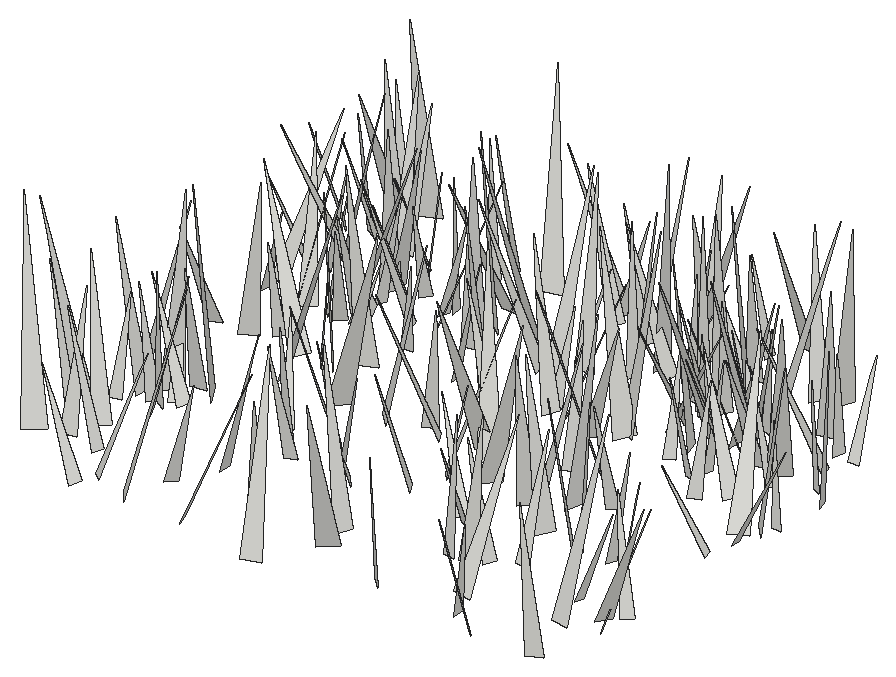
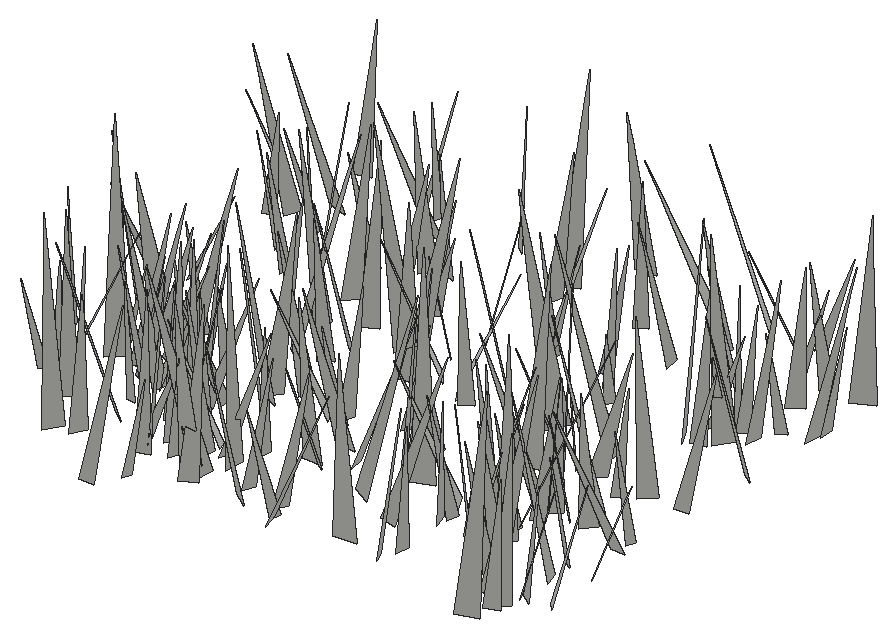
# SketchUp Ruby script. Lengths in inches.
U = 1.inch
M = Sketchup.active_model
def pt(a) = Geom::Point3d.new(a.map { |v| v * U })
def face(e, loops, mat)
  f = e.add_face(loops[0].map { |a| pt(a) })
  loops[1..].each { |l| e.add_face(l.map { |a| pt(a) }).erase! }
  f.material = f.back_material = mat if mat
  f
end
# faces: each face lists its corners as indices into pts; further lists are holes
def faces(e, pts, list, mat = nil) = list.each { |f| face(e, (f[0].is_a?(Array) ? f : [f]).map { |l| l.map { |i| pts[i] } }, mat) }
# xy, xz, yz: faces in a plane at the given z, y or x. An outline is a flat list of corners, or four numbers for a rectangle; further outlines are holes
def ring(l) = l.size == 4 ? [[l[0], l[1]], [l[2], l[1]], [l[2], l[3]], [l[0], l[3]]] : l.each_slice(2).to_a
def flat(e, list, mat, &to3) = list.each { |f| face(e, (f[0].is_a?(Array) ? f : [f]).map { |l| ring(l).map { |u, v| to3.(u, v) } }, mat) }
def xy(e, z, list, mat = nil) = flat(e, list, mat) { |x, y| [x, y, z] }
def xz(e, y, list, mat = nil) = flat(e, list, mat) { |x, z| [x, y, z] }
def yz(e, x, list, mat = nil) = flat(e, list, mat) { |y, z| [x, y, z] }
def lines(e, pts, list) = list.each { |a, b| e.add_line(pt(pts[a]), pt(pts[b])) }
# prism: a flat outline (further loops are holes) pulled along v
def prism(e, loops, v, mat = nil)
  f = face(e, loops, mat); d = Geom::Vector3d.new(v.map { |x| x * U })
  f.pushpull(f.normal.samedirection?(d) ? d.length : -d.length)
end
def box(e, o, s, mat = nil) = prism(e, [[o, [o[0] + s[0], o[1], o[2]], [o[0] + s[0], o[1] + s[1], o[2]], [o[0], o[1] + s[1], o[2]]]], [0, 0, s[2]], mat)
def at(x, y, z, deg = 0) = Geom::Transformation.translation(pt([x, y, z])) * Geom::Transformation.rotation(ORIGIN, Z_AXIS, deg.degrees)
def axes(o, x, y, z) = Geom::Transformation.new([*x, 0, *y, 0, *z, 0, *pt(o).to_a, 1])
def part(name) = M.definitions.add(name)
# library, detail: a bought-in or finely detailed component or shape, given as its bounding box
def library(name, o, s) = part(name).tap { |d| box(d.entities, o, s) }
def detail(e, o, s) = box(e.add_group.entities, o, s)
def put(e, d, t, mat = nil) = e.add_instance(d, t).tap { |i| i.material = mat if mat }
def group(e, t, mat = nil) = e.add_group.tap { |g| g.transformation = t; g.material = mat if mat }.entities
root = M.entities
c1 = part("fur_instance\#9")
p = [[0.8125,0,1.79],[0.67,-0.02,1.48],[0,-0.11,0],[0,0.11,0]]
faces(c1.entities,p,[[0,1,2,3]])
put(root,c1,axes([494.74,158.14,-21.66],[-2.89308,-3.13599,0.85003],[-3.23039,2.89836,-0.3018],[0.34876,0.83187,4.25597]))
put(root,c1,axes([462.16,157.61,-21.66],[-3.83694,1.86592,0.39498],[1.90547,3.78872,0.61201],[0.08273,-0.72368,4.22246]))
put(root,c1,axes([500.03,158.27,-21.66],[1.93856,-5.12728,2.24723],[-5.46022,-2.25638,-0.43794],[-1.23493,1.9279,5.46399]))
put(root,c1,axes([477.57,156.7,-21.66],[-1.40207,7.22786,1.13046],[7.31414,1.36087,0.37039],[-0.15287,-1.17973,7.35327]))
put(root,c1,axes([485.84,159.52,-21.66],[-2.86919,-3.90872,1.79506],[-4.01549,3.2075,0.56601],[1.54149,1.08002,4.8156]))
put(root,c1,axes([480.32,161.42,-21.66],[4.1786,-6.03386,0.40804],[-6.0035,-4.19846,-0.60465],[-0.72937,-0.01047,7.31455]))
put(root,c1,axes([492.57,159.67,-21.66],[3.92592,-0.41216,0.89749],[-0.2951,-4.00034,-0.54626],[-0.94248,-0.46433,3.90952]))
put(root,c1,axes([470.65,158.23,-21.66],[5.67742,2.27779,0.25934],[2.25803,-5.67581,0.41845],[-0.39608,0.29237,6.10297]))
put(root,c1,axes([465.71,158.26,-21.66],[6.07013,4.91373,1.22638],[4.90353,-6.18107,0.495],[-1.26656,-0.38061,7.79399]))
put(root,c1,axes([462.77,159.21,-21.66],[2.99625,3.60782,0.19235],[3.59342,-3.00177,0.328],[-0.37513,0.06212,4.67828]))
put(root,c1,axes([466.91,161.75,-21.66],[3.70766,-2.56946,0.56874],[-2.62102,-3.69364,0.39947],[-0.23628,0.65362,4.49325]))
put(root,c1,axes([473.18,162.7,-21.66],[1.74282,-4.6233,0.69197],[-4.67126,-1.6936,0.44965],[0.18179,0.80496,4.92038]))
put(root,c1,axes([460.64,161.9,-21.66],[-4.9286,0.63717,0.02707],[0.62924,4.89286,-0.60144],[0.10377,0.59304,4.93308]))
put(root,c1,axes([455.53,161.61,-21.66],[-4.19179,6.94453,1.88873],[7.18228,4.17546,0.58769],[0.45687,-1.92457,8.09026]))
put(root,c1,axes([457.78,162.37,-21.66],[-1.16882,5.10436,1.64073],[5.31118,1.33199,-0.3603],[0.7334,-1.51127,5.22406]))
put(root,c1,axes([491.24,161.73,-21.66],[0.40052,6.46259,0.29319],[6.45769,-0.38185,-0.40475],[0.38629,-0.31712,6.46233]))
put(root,c1,axes([500.51,164.9375,-21.66],[5.28357,-2.5058,0.04843],[-2.504,-5.27298,0.35108],[0.10676,0.33794,5.83712]))
put(root,c1,axes([479.9,163.52,-21.66],[-6.40273,2.01611,1.14645],[1.98655,6.50456,-0.34415],[1.19695,-0.01086,6.70383]))
put(root,c1,axes([501.34,163.74,-21.66],[4.04394,2.43918,0.42992],[2.39305,-4.06014,0.52577],[-0.63852,0.23141,4.69325]))
put(root,c1,axes([498.6,162.74,-21.66],[1.7832,7.11152,0.69499],[7.11724,-1.83129,0.47737],[-0.63379,-0.55606,7.31612]))
put(root,c1,axes([458.62,164.75,-21.66],[3.00603,-4.02582,3.59921],[-4.80148,-3.87769,-0.32715],[-2.47129,2.63706,5.01362]))
put(root,c1,axes([488.66,165.64,-21.66],[3.55242,-4.27149,1.91187],[-4.60398,-3.6203,0.46613],[-0.83917,1.77997,5.53606]))
put(root,c1,axes([468.61,165.19,-21.66],[5.20805,0.62891,1.21236],[0.54515,-5.33937,0.42794],[-1.25226,0.29119,5.2284]))
put(root,c1,axes([487.3125,165.27,-21.66],[1.36793,4.62634,1.5435],[4.80198,-1.5578,0.41343],[-0.85231,-1.35162,4.8066]))
put(root,c1,axes([497.63,166.01,-21.66],[3.74369,-0.67268,0.40161],[-0.71907,-3.7286,0.45768],[-0.31101,0.52348,3.776]))
put(root,c1,axes([489.94,166.25,-21.66],[-4.10178,1.61092,0.95507],[1.70987,4.15942,0.32775],[0.76391,-0.66031,4.39457]))
put(root,c1,axes([501.63,166.01,-21.66],[-2.18486,3.79279,1.02862],[3.92891,2.13324,0.47945],[0.08359,-1.13179,4.35074]))
put(root,c1,axes([454.9,166.18,-21.66],[-4.79431,0.50788,0.77321],[0.45097,4.84644,-0.38709],[0.80772,0.30866,4.80557]))
put(root,c1,axes([455.1,167.34,-21.66],[-7.08698,0.49693,1.41438],[0.58095,7.2106,0.37757],[1.38199,-0.48283,7.09434]))
put(root,c1,axes([485.54,169.17,-21.66],[-1.12897,-3.54048,0.33773],[-3.515,1.16474,0.46018],[0.54205,0.17891,3.68752]))
put(root,c1,axes([471.09,168.99,-21.66],[0.8668,-4.44855,1.11397],[-4.54098,-0.99091,-0.42373],[-0.6404,1.00517,4.51236]))
put(root,c1,axes([476.07,169.02,-21.66],[-5.08924,-4.37631,0.84531],[-4.44671,5.07308,-0.50754],[0.30556,0.93743,6.69289]))
put(root,c1,axes([491.84,167.27,-21.66],[-0.34341,4.80516,0.97397],[4.88667,0.41477,-0.32328],[0.39826,-0.94579,4.80656]))
put(root,c1,axes([460.12,168.19,-21.66],[5.04239,2.3615,1.06864],[2.46365,-5.09289,-0.37039],[-0.80566,-0.79378,5.55564]))
put(root,c1,axes([457.17,168.06,-21.66],[-1.25475,3.57203,1.31412],[3.70812,1.4592,-0.42579],[0.858,-1.08261,3.76198]))
put(root,c1,axes([494.96,168.99,-21.66],[-5.04486,-3.51647,1.75014],[-3.733,5.17856,-0.35556],[1.22196,1.30239,6.1392]))
put(root,c1,axes([475.125,169.16,-21.66],[4.21688,0.53755,0.91963],[0.65776,-4.26755,-0.52159],[-0.83787,-0.64478,4.21888]))
put(root,c1,axes([459.24,169.4375,-21.66],[-3.39336,2.50243,2.08506],[2.97495,3.60715,0.51243],[1.32637,-1.68843,4.18502]))
put(root,c1,axes([459.875,169.29,-21.66],[-2.18081,-4.36379,1.96245],[-4.63729,2.45895,0.31456],[1.17875,1.60022,4.86823]))
put(root,c1,axes([498.56,169.11,-21.66],[3.70099,1.78589,1.07617],[1.91017,-3.78303,-0.29128],[-0.83593,-0.7377,4.09901]))
put(root,c1,axes([475.42,169.16,-21.66],[-4.70558,-0.80345,0.83315],[-0.88013,4.74917,-0.39105],[0.7517,0.53106,4.75763]))
put(root,c1,axes([469.64,170.53,-21.66],[-0.67343,-4.75938,1.30258],[-4.88536,0.82798,0.49956],[0.69398,1.21023,4.78075]))
put(root,c1,axes([479.72,170.8,-21.66],[-3.92886,-2.51502,0.86647],[-2.44083,4.02285,0.60923],[1.05758,-0.05874,4.62495]))
put(root,c1,axes([458,169.93,-21.66],[-6.22894,0.57755,1.75246],[0.68588,6.45268,0.31131],[1.71297,-0.48351,6.24791]))
put(root,c1,axes([461.21,170.1875,-21.66],[-4.19942,1.95994,0.17006],[1.96728,4.18576,0.33862],[0.01038,-0.37878,4.62189]))
put(root,c1,axes([484.73,169.93,-21.66],[-3.18645,2.79123,0.05753],[2.78151,3.16651,0.42911],[-0.23972,-0.36053,4.21429]))
put(root,c1,axes([460.53,172.53,-21.66],[1.15457,-5.41906,0.82486],[-5.48032,-1.12384,0.28761],[0.11275,0.86626,5.53322]))
put(root,c1,axes([490.32,171.58,-21.66],[-5.43342,3.18473,2.47254],[3.60205,5.6984,0.57576],[1.81141,-1.77869,6.27161]))
put(root,c1,axes([459.32,171.35,-21.66],[6.01123,-4.10409,2.83515],[-4.50522,-6.3728,0.32708],[-2.14119,1.8869,7.27128]))
put(root,c1,axes([496.09,171.28,-21.66],[4.13039,-0.87619,1.21239],[-0.99071,-4.26996,0.28929],[-1.12075,0.54542,4.21238]))
put(root,c1,axes([493.3,171.625,-21.66],[-3.24328,-4.06122,2.56752],[-4.33534,3.80899,0.54855],[2.07134,1.61325,5.16831]))
put(root,c1,axes([460.5,170.14,-21.66],[-2.92778,3.00983,0.00711],[2.98882,2.90849,-0.48849],[0.35507,0.33555,4.17041]))
put(root,c1,axes([461.84,172.41,-21.66],[-6.4664,-4.252,2.80304],[-4.40658,6.94256,0.3657],[2.55316,1.21333,7.73047]))
put(root,c1,axes([487.1,173.8125,-21.66],[3.86717,-5.0611,1.49434],[-5.13106,-4.03908,-0.40116],[-1.23289,0.93486,6.35679]))
put(root,c1,axes([468.5,171.88,-21.66],[-2.98771,2.56269,0.00271],[2.54357,2.96592,-0.47684],[0.31249,0.36018,3.90722]))
put(root,c1,axes([483.3125,174.62,-21.66],[6.15872,-4.73604,0.69713],[-4.78091,-6.14284,0.50431],[-0.2428,0.82545,7.75278]))
put(root,c1,axes([480.49,173.51,-21.66],[2.6007,2.51832,0.88377],[2.64819,-2.58836,-0.41733],[-0.33183,-0.9193,3.59603]))
put(root,c1,axes([455.1875,174.09,-21.66],[3.97347,4.57155,1.31094],[4.73936,-3.94824,-0.59665],[-0.39506,-1.38509,6.02757]))
put(root,c1,axes([480.45,177.76,-21.66],[1.9178,-7.47283,0.23219],[-7.45531,-1.92947,-0.52008],[-0.56157,0.09505,7.69744]))
put(root,c1,axes([500.375,175.97,-21.66],[-3.53813,-0.73541,0.01575],[-0.72603,3.50386,0.50526],[0.11809,-0.49152,3.57826]))
put(root,c1,axes([469.12,176.52,-21.66],[6.86151,-4.43995,0.81428],[-4.49635,-6.85344,0.51929],[-0.39875,0.87961,8.15621]))
put(root,c1,axes([489.57,175.5,-21.66],[6.98669,-0.82296,2.45735],[-1.02769,-7.36659,0.45485],[-2.37901,0.76535,7.02027]))
put(root,c1,axes([491.78,176.87,-21.66],[1.41164,-4.04262,0.99191],[-4.10193,-1.52908,-0.39425],[-0.70768,0.79907,4.26381]))
put(root,c1,axes([476.96,177.23,-21.66],[-4.6266,-2.97065,0.07987],[-2.96143,4.59663,-0.58091],[-0.24706,0.53178,5.46742]))
put(root,c1,axes([475.66,177.875,-21.66],[2.40691,-4.24835,1.2679],[-4.42272,-2.4014,0.34948],[-0.30924,1.27831,4.87028]))
put(root,c1,axes([488.72,179.57,-21.66],[-4.98525,-6.36904,1.05647],[-6.36247,5.07321,0.56124],[1.09531,0.48105,8.06861]))
put(root,c1,axes([463.77,177.42,-21.66],[7.81228,1.65656,1.00866],[1.73052,-7.84393,-0.52089],[-0.87571,-0.72239,7.96898]))
put(root,c1,axes([472.59,176.87,-21.66],[4.81614,4.80746,1.57054],[5.00941,-4.83285,-0.56818],[-0.69571,-1.51836,6.78115]))
put(root,c1,axes([486.0625,176.92,-21.66],[3.37327,4.28522,1.21914],[4.44713,-3.33099,-0.5966],[-0.2692,-1.33033,5.4209]))
put(root,c1,axes([479.08,176.04,-21.66],[4.55508,3.875,0.43107],[3.83788,-4.57312,0.55448],[-0.68713,0.14532,5.95457]))
put(root,c1,axes([481.54,176.73,-21.66],[-3.76745,6.43232,1.47995],[6.58457,3.78058,0.33053],[0.45645,-1.44608,7.44709]))
put(root,c1,axes([455.9,180.1,-21.66],[1.11267,-4.69864,0.20362],[-4.67497,-1.12782,-0.47895],[-0.51316,0.0867,4.80478]))
put(root,c1,axes([500.875,178.27,-21.66],[4.1398,0.29454,0.02134],[0.28882,-4.10074,0.57065],[-0.06159,0.56772,4.11084]))
put(root,c1,axes([486.46,179.08,-21.66],[-2.20726,4.7722,2.01563],[5.04733,2.47451,-0.33147],[1.16667,-1.67676,5.24748]))
put(root,c1,axes([458.67,180.17,-21.66],[3.92094,-4.8226,1.73149],[-5.06492,-3.97791,0.39007],[-0.77596,1.59628,6.20315]))
put(root,c1,axes([464.8,180,-21.66],[2.81827,1.89164,1.24112],[2.11841,-2.90244,-0.38665],[-0.79437,-1.02901,3.37216]))
put(root,c1,axes([465.55,180.36,-21.66],[4.83002,3.67653,3.08875],[4.26917,-5.29337,-0.3752],[-2.19806,-2.20219,6.05848]))
put(root,c1,axes([467.53,178.52,-21.66],[2.30646,3.84948,0.31393],[3.83736,-2.32546,0.32205],[-0.43787,-0.10267,4.47599]))
put(root,c1,axes([460.3,181.34,-21.66],[2.53184,-2.74895,1.13947],[-2.76231,-2.72751,-0.44237],[-1.1067,0.51894,3.71097]))
put(root,c1,axes([501.12,180.51,-21.66],[4.60486,4.04407,1.88978],[4.30358,-4.74303,-0.33665],[-1.18533,-1.50984,6.1193]))
put(root,c1,axes([467.27,181.7,-21.66],[-2.10134,6.53759,3.4605],[7.38552,2.05442,0.60354],[0.41142,-3.48856,6.84043]))
put(root,c1,axes([462.99,180.08,-21.66],[-5.62336,3.63446,0.06059],[3.63174,5.6129,0.37548],[-0.15301,-0.3482,6.6851]))
put(root,c1,axes([495.02,181.27,-21.66],[2.53545,-3.02814,1.98338],[-3.53036,-2.60371,0.53779],[-0.80002,1.89288,3.91266]))
put(root,c1,axes([501.8,181.4,-21.66],[0.50374,3.60666,1.32904],[3.78488,-0.69911,0.46265],[-0.67011,-1.23747,3.61216]))
put(root,c1,axes([500.32,179.31,-21.66],[-3.69849,5.78351,0.10997],[5.76561,3.69627,-0.48502],[0.46777,0.16892,6.84781]))
put(root,c1,axes([484.59,183.28,-21.66],[4.6953,-3.04636,0.27903],[-3.0591,-4.67738,0.40996],[-0.01004,0.49581,5.58194]))
put(root,c1,axes([476.62,182.77,-21.66],[-3.90024,1.94852,0.94584],[2.05782,3.9414,0.36592],[0.67579,-0.75618,4.3445]))
put(root,c1,axes([493.02,183.24,-21.66],[-1.62958,-3.15436,1.09529],[-3.33909,1.53504,-0.54711],[-0.01197,1.22427,3.50802]))
put(root,c1,axes([496.92,182.78,-21.66],[-4.22119,3.06488,0.48562],[3.10212,4.18863,0.52921],[0.07866,-0.71394,5.1896]))
put(root,c1,axes([462.11,185.41,-21.66],[3.06057,-3.28635,0.3748],[-3.27189,-3.08287,-0.31361],[-0.4851,0.05914,4.47983]))
put(root,c1,axes([467.99,185.02,-21.66],[1.46502,-3.697,0.60293],[-3.73698,-1.39797,0.50827],[0.25762,0.74531,3.94408]))
put(root,c1,axes([494.71,185.4375,-21.66],[-1.89303,-4.40404,0.51291],[-4.43222,1.86471,-0.34716],[-0.11875,0.60786,4.78107]))
put(root,c1,axes([474.66,184.68,-21.66],[-6.1633,-1.76581,2.36846],[-1.74431,6.59751,0.37966],[2.38433,0.26209,6.40002]))
put(root,c1,axes([472.91,183.96,-21.66],[4.24313,0.45781,1.20359],[0.34307,-4.39664,0.46288],[-1.24117,0.34981,4.24258]))
put(root,c1,axes([459.26,184.1,-21.66],[6.44327,3.68852,1.42181],[3.82977,-6.4983,-0.49739],[-0.97955,-1.14429,7.40767]))
put(root,c1,axes([497.5625,187.03,-21.66],[5.80631,-5.6916,0.53269],[-5.68589,-5.82856,-0.29992],[-0.59055,0.15799,8.12513]))
put(root,c1,axes([493.5625,184.5625,-21.66],[3.9323,-0.29865,1.47953],[-0.48436,-4.16008,0.44758],[-1.42954,0.58799,3.91814]))
put(root,c1,axes([486.43,184.8,-21.66],[5.34271,-3.44394,4.19103],[-3.85612,-6.54857,-0.46545],[-3.8152,1.796,6.33945]))
put(root,c1,axes([455.6875,185.67,-21.66],[3.70802,-0.97097,0.29213],[-0.94384,-3.70994,-0.3508],[-0.37053,-0.26665,3.81695]))
put(root,c1,axes([490.47,184.37,-21.66],[-2.63101,2.88231,1.12737],[2.88894,2.81797,-0.46255],[1.11028,-0.50218,3.87505]))
put(root,c1,axes([480.58,184.3,-21.66],[-5.69821,2.17721,0.97614],[2.15034,5.78116,-0.34192],[1.034,-0.02439,6.0904]))
put(root,c1,axes([491.45,187.97,-21.66],[-1.56855,-7.63886,0.47282],[-7.63369,1.59619,0.46371],[0.55001,0.36889,7.78444]))
put(root,c1,axes([462.4,186.98,-21.66],[2.27929,-4.31761,0.37807],[-4.29346,-2.30768,-0.46977],[-0.59235,0.11282,4.85966]))
put(root,c1,axes([495.66,187.22,-21.66],[1.37303,-5.10418,0.31363],[-5.09334,-1.39399,-0.38851],[-0.45708,0.20095,5.27134]))
put(root,c1,axes([480.3,185.16,-21.66],[1.50954,-3.07856,1.78204],[-3.55315,-1.39659,0.59714],[-0.16832,1.87187,3.37633]))
put(root,c1,axes([463.09,187.68,-21.66],[-6.90561,-3.33755,0.10935],[-3.32242,6.89219,0.54573],[0.33571,-0.44394,7.65042]))
put(root,c1,axes([481.64,184.7,-21.66],[4.67763,2.46387,0.32375],[2.42875,-4.67875,0.51598],[-0.52599,0.30722,5.26162]))
put(root,c1,axes([486.12,185.34,-21.66],[3.51282,6.48869,2.15536],[6.79895,-3.57131,-0.32959],[-0.72316,-2.057,7.37118]))
put(root,c1,axes([497.94,185.59,-21.66],[-4.0966,0.35691,0.30901],[0.31396,4.07547,-0.54495],[0.35257,0.51784,4.07585]))
put(root,c1,axes([502.125,185.8,-21.66],[-4.83531,-1.63891,2.39644],[-2.01972,5.24312,-0.48946],[2.08559,1.27782,5.08199]))
put(root,c1,axes([460.95,185.48,-21.66],[3.02903,2.92229,1.12241],[2.89072,-3.2105,0.55771],[-1.2014,-0.35704,4.17178]))
put(root,c1,axes([471.37,187.83,-21.66],[2.47243,-7.62212,2.09201],[-7.90302,-2.41845,0.52868],[-0.12434,2.1542,7.99563]))
put(root,c1,axes([490.65,186.4375,-21.66],[-6.07164,-2.28107,2.04855],[-2.55827,6.27412,-0.5961],[1.68971,1.3026,6.45854]))
put(root,c1,axes([488.82,188.46,-21.66],[-1.13114,-4.608,0.05517],[-4.59723,1.12439,-0.34274],[-0.31976,0.13515,4.73241]))
put(root,c1,axes([459.23,185.6,-21.66],[-4.06626,4.25963,1.22614],[4.27905,4.20638,-0.4224],[1.15655,-0.5867,5.87371]))
put(root,c1,axes([466.35,187.64,-21.66],[-5.39834,-1.72938,0.70035],[-1.70183,5.44274,0.32197],[0.76486,-0.09564,5.65943]))
put(root,c1,axes([462.7,186.06,-21.66],[6.72772,1.76518,0.89994],[1.69777,-6.77807,0.60273],[-1.02144,0.36032,6.92927]))
put(root,c1,axes([500.65,187.03,-21.66],[1.66971,3.21733,1.57549],[3.35444,-2.01427,0.55833],[-1.25742,-1.10127,3.58153]))
put(root,c1,axes([494.3,188.49,-21.66],[-2.38494,-6.16406,1.52656],[-6.35023,2.30898,-0.59758],[-0.0234,1.63919,6.58229]))
put(root,c1,axes([492.99,188.4,-21.66],[-3.34237,-3.67886,0.49489],[-3.71061,3.29315,-0.58039],[-0.10119,0.75599,4.93646]))
put(root,c1,axes([494.91,188.03,-21.66],[-3.3946,-3.12525,1.18102],[-3.29173,3.41661,-0.4203],[0.5714,1.11577,4.59499]))
put(root,c1,axes([476.3125,188.5625,-21.66],[-6.23663,-1.3966,0.55844],[-1.37103,6.25805,0.33911],[0.61857,-0.21031,6.38209]))
put(root,c1,axes([488.09,187.5,-21.66],[4.49912,0.07902,0.02983],[0.07502,-4.46879,0.52292],[-0.03881,0.52233,4.46932]))
put(root,c1,axes([465.27,189.02,-21.66],[-3.54687,-2.63553,0.56126],[-2.61948,3.58991,0.30355],[0.63194,0.08835,4.40842]))
put(root,c1,axes([492.67,188.63,-21.66],[6.50661,-0.43072,0.76621],[-0.39332,-6.54513,-0.33931],[-0.78607,-0.29036,6.51202]))
put(root,c1,axes([499.53,189.4,-21.66],[-5.35424,-1.86738,0.02315],[-1.86377,5.3475,0.29345],[0.11847,-0.26947,5.66294]))
put(root,c1,axes([462.74,188.84,-21.66],[4.01633,-1.15722,1.23996],[-1.33038,-4.12648,0.45808],[-1.05202,0.80037,4.15454]))
put(root,c1,axes([455.75,186.92,-21.66],[1.29367,6.30142,0.29631],[6.29029,-1.26564,-0.54746],[0.47747,-0.39942,6.4095]))
put(root,c1,axes([484.34,188.2,-21.66],[4.33311,5.30156,2.10924],[5.44411,-4.63436,0.46433],[-1.70794,-1.32191,6.83131]))
put(root,c1,axes([462.28,190.43,-21.66],[5.8288,-3.89293,1.62458],[-3.86791,-6.0381,-0.59132],[-1.68328,0.3943,6.98428]))
put(root,c1,axes([494.07,188.62,-21.66],[4.8135,2.02359,1.54657],[1.94555,-5.05552,0.55956],[-1.64367,-0.05793,5.19149]))
put(root,c1,axes([488.74,189.91,-21.66],[-0.48959,-3.44443,1.08487],[-3.54488,0.6673,0.51889],[0.68909,0.98557,3.44014]))
put(root,c1,axes([478.3125,187.2,-21.66],[0.44326,7.59594,0.73525],[7.62112,-0.4789,0.35297],[-0.39679,-0.71255,7.60067]))
put(root,c1,axes([454.78,190.74,-21.66],[-3.14416,-1.79317,0.28571],[-1.75542,3.14785,0.43854],[0.46429,-0.24163,3.59289]))
put(root,c1,axes([467.79,188.38,-21.66],[5.23362,2.8594,0.35445],[2.818,-5.23298,0.60609],[-0.60055,0.36375,5.93293]))
put(root,c1,axes([488.49,190.79,-21.66],[-4.19066,-2.50752,1.09961],[-2.47633,4.32875,0.43379],[1.16817,0.18082,4.86427]))
put(root,c1,axes([473.5,191.58,-21.66],[-3.27464,-6.78559,1.40651],[-6.92909,3.22889,-0.5548],[0.10135,1.50857,7.51397]))
put(root,c1,axes([466.92,190.2,-21.66],[4.20297,-1.11156,0.80651],[-1.18233,-4.24977,0.30429],[-0.69867,0.5049,4.33681]))
put(root,c1,axes([464.49,191.37,-21.66],[2.8154,-3.04723,0.70248],[-2.99803,-2.89898,-0.55973],[-0.88933,0.126,4.11081]))
put(root,c1,axes([462.32,191.14,-21.66],[6.13982,-1.63324,0.91897],[-1.58888,-6.20592,-0.4139],[-0.99371,-0.16841,6.33984]))
put(root,c1,axes([457.17,190.38,-21.66],[2.36922,2.94645,1.17355],[3.15581,-2.33594,-0.5062],[-0.31572,-1.23846,3.7468]))
put(root,c1,axes([489.5,191.42,-21.66],[-3.20699,2.34244,2.63387],[2.95903,3.72406,0.29089],[1.91533,-1.83124,3.96071]))
put(root,c1,axes([470.85,190.71,-21.66],[3.81307,5.29138,3.34018],[5.75803,-4.49829,0.55278],[-2.44962,-2.33704,6.49867]))
put(root,c1,axes([493.15,191.125,-21.66],[-0.92871,-3.83483,1.6083],[-4.04735,1.2119,0.55253],[0.95473,1.40727,3.90681]))
put(root,c1,axes([488.53,190.37,-21.66],[1.00735,6.64791,2.58508],[7.07427,-1.26504,0.49655],[-0.91221,-2.46923,6.70544]))
put(root,c1,axes([477.91,190.35,-21.66],[2.28219,3.09258,0.57784],[3.14608,-2.24088,-0.43237],[0.01087,-0.72161,3.81909]))
put(root,c1,axes([469.91,193.28,-21.66],[-0.6438,-6.00502,0.1729],[-5.98541,0.62626,-0.53591],[-0.51472,0.22839,6.0156]))
put(root,c1,axes([486.6,191.375,-21.66],[0.02782,-4.7345,1.86898],[-5.06027,0.17616,0.52158],[0.54982,1.86087,4.70577]))
put(root,c1,axes([478.82,190,-21.66],[-0.28002,6.79198,1.74012],[7.00527,0.19856,0.35229],[-0.29175,-1.75129,6.78861]))
put(root,c1,axes([498.79,191.66,-21.66],[3.6892,-1.49713,1.29137],[-1.47127,-3.90506,-0.32413],[-1.32076,0.16824,3.96818]))
put(root,c1,axes([467.3,191.02,-21.66],[-4.422,-0.95671,1.75223],[-1.16644,4.69405,-0.38074],[1.6202,0.76828,4.50826]))
put(root,c1,axes([464.14,191.87,-21.66],[3.95435,2.54343,1.52337],[2.80761,-4.0284,-0.56212],[-0.95239,-1.31514,4.66797]))
put(root,c1,axes([481.83,191.375,-21.66],[-5.13165,1.21269,1.54361],[1.09048,5.35359,-0.58061],[1.63224,0.23592,5.24093]))
put(root,c1,axes([496.68,193.13,-21.66],[2.3512,-5.85332,1.44977],[-6.03015,-2.28819,0.5412],[-0.02311,1.54732,6.28463]))
put(root,c1,axes([500.26,191.375,-21.66],[-0.72601,3.76819,0.7458],[3.80081,0.81458,-0.41575],[0.55615,-0.64789,3.8149]))
put(root,c1,axes([484.77,192.07,-21.66],[4.2362,2.18763,0.04516],[2.18011,-4.21144,-0.49393],[0.18673,-0.4595,4.74206]))
put(root,c1,axes([456.86,192.49,-21.66],[6.14666,2.4589,1.36982],[2.59506,-6.2248,-0.47069],[-1.09008,-0.95377,6.60349]))
put(root,c1,axes([487.59,193.53,-21.66],[6.10585,-2.9623,2.45846],[-2.96929,-6.55789,-0.52733],[-2.45002,0.56525,6.76598]))
put(root,c1,axes([483.79,192.88,-21.66],[-5.48132,1.03762,0.48302],[1.07413,5.47965,0.41785],[0.39525,-0.50168,5.563]))
put(root,c1,axes([484.78,193.45,-21.66],[5.5976,-0.64404,1.05715],[-0.59203,-5.69245,-0.3332],[-1.08713,-0.21617,5.62467]))
put(root,c1,axes([462.17,194.6,-21.66],[-2.39227,-3.29447,0.41561],[-3.24315,2.42809,0.57931],[0.71291,-0.00928,4.03]))
put(root,c1,axes([482.44,193.68,-21.66],[7.55648,0.00384,2.83421],[0.13477,-8.06186,-0.34839],[-2.831,-0.37353,7.54844]))
put(root,c1,axes([458.66,196.58,-21.66],[1.6119,-7.35068,0.1441],[-7.34568,-1.61634,-0.28263],[-0.30696,0.08011,7.52003]))
put(root,c1,axes([454.56,195.375,-21.66],[-3.11694,-3.18155,0.61605],[-3.14817,3.17551,0.47138],[0.76862,0.10457,4.42892]))
put(root,c1,axes([489.18,194.54,-21.66],[-3.99444,1.28958,0.25526],[1.31279,3.95594,0.55757],[0.06915,-0.60932,4.16025]))
put(root,c1,axes([456.87,195.68,-21.66],[-3.51503,-1.89548,0.64915],[-1.82323,3.56963,0.55065],[0.83071,-0.18586,3.95538]))
put(root,c1,axes([488.67,194.74,-21.66],[-5.61783,-2.93903,2.21928],[-3.25584,5.85535,-0.48739],[1.72124,1.48327,6.32142]))
put(root,c1,axes([460.72,193.07,-21.66],[-0.70792,6.63222,0.94241],[6.69223,0.65809,0.39581],[-0.29764,-0.97786,6.65814]))
put(root,c1,axes([488.2,196.13,-21.66],[1.13187,-5.42392,1.09616],[-5.52646,-1.05128,0.50466],[0.2806,1.17367,5.51773]))
put(root,c1,axes([492.6,193.19,-21.66],[4.44163,5.80553,0.93246],[5.82565,-4.50337,0.28854],[-0.79717,-0.56325,7.30404]))
put(root,c1,axes([479.85,195.43,-21.66],[-4.92159,1.07561,1.43405],[1.22896,5.07505,0.41117],[1.30503,-0.72281,5.02095]))
put(root,c1,axes([456.39,195.71,-21.66],[-2.19445,-3.56039,1.55722],[-3.85398,2.22319,-0.34801],[0.4981,1.5159,4.16783]))
put(root,c1,axes([483.5,197.16,-21.66],[3.36896,-5.0045,1.18358],[-5.04079,-3.49374,-0.42432],[-1.01802,0.73793,6.01788]))
put(root,c1,axes([459.9,195,-21.66],[-0.06431,5.36711,1.48252],[5.54585,0.19413,-0.46222],[0.49719,-1.47116,5.34755]))
put(root,c1,axes([466.83,195.62,-21.66],[-4.7956,1.01448,1.55419],[0.95492,5.04106,-0.34401],[1.59148,0.0322,4.88965]))
put(root,c1,axes([486.3,194.98,-21.66],[-4.11869,2.39634,0.55767],[2.352,4.15398,-0.47915],[0.72219,0.13795,4.74094]))
put(root,c1,axes([483.18,195.96,-21.66],[7.44021,-1.05618,0.97458],[-1.13327,-7.472,0.55406],[-0.88376,0.68976,7.49435]))
put(root,c1,axes([494.86,197.07,-21.66],[6.65936,-3.07974,1.86174],[-3.09449,-6.89952,-0.34452],[-1.83712,0.458,7.32893]))
put(root,c1,axes([476.62,196.14,-21.66],[-5.29366,2.0126,1.17564],[2.12712,5.36423,0.39489],[0.95291,-0.79376,5.64955]))
put(root,c1,axes([467.46,197.25,-21.66],[-4.6895,-2.45579,1.69505],[-2.43913,4.97359,0.45768],[1.71894,0.35769,5.27378]))
put(root,c1,axes([484.01,196.1875,-21.66],[-2.76968,5.79414,2.34049],[6.07448,3.09716,-0.47899],[1.46654,-1.88589,6.4042]))
put(root,c1,axes([457.16,197.35,-21.66],[-4.56803,3.68378,2.77525],[4.20348,4.93276,0.37129],[1.89817,-2.05836,5.85656]))
put(root,c1,axes([493.25,196.47,-21.66],[-5.08391,3.17186,1.29588],[3.17676,5.23223,-0.34381],[1.28383,-0.38638,5.98237]))
put(root,c1,axes([476.11,197.32,-21.66],[3.72364,-1.08643,0.80362],[-1.21362,-3.72465,0.58799],[-0.59435,0.79892,3.83407]))
put(root,c1,axes([476.02,197.94,-21.66],[-5.88175,-1.50758,0.15009],[-1.51502,5.85044,-0.60606],[-0.00586,0.62434,6.04156]))
put(root,c1,axes([470.67,196.83,-21.66],[-1.87564,7.62096,1.95831],[7.8685,1.80971,0.49369],[-0.027,-2.0194,7.83284]))
put(root,c1,axes([457.38,198.07,-21.66],[1.73924,-4.25815,2.51532],[-4.74882,-2.1825,-0.41111],[-1.38108,2.14207,4.58125]))
put(root,c1,axes([479.3125,196.93,-21.66],[3.26782,5.25044,1.3347],[5.28581,-3.43164,0.55786],[-1.18691,-0.82697,6.1591]))
put(root,c1,axes([458.09,199.78,-21.66],[2.83404,-7.21043,2.36501],[-7.48804,-3.06648,-0.37599],[-1.22999,2.05469,7.73827]))
put(root,c1,axes([487.07,199.11,-21.66],[-3.6032,0.74818,1.09352],[0.87855,3.72087,0.34907],[0.99182,-0.57787,3.66346]))
put(root,c1,axes([488.7,201.36,-21.66],[-0.42981,-6.03201,0.26249],[-6.01913,0.44871,0.45551],[0.47339,0.22867,6.03012]))
